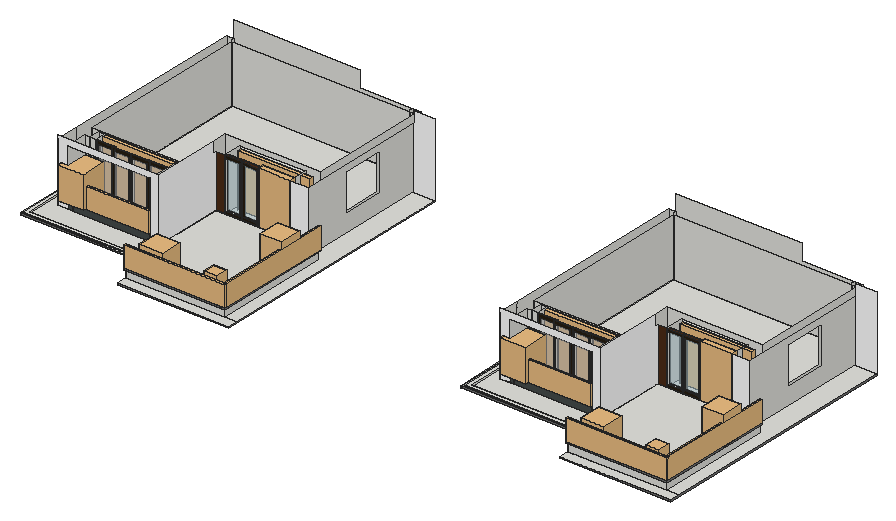
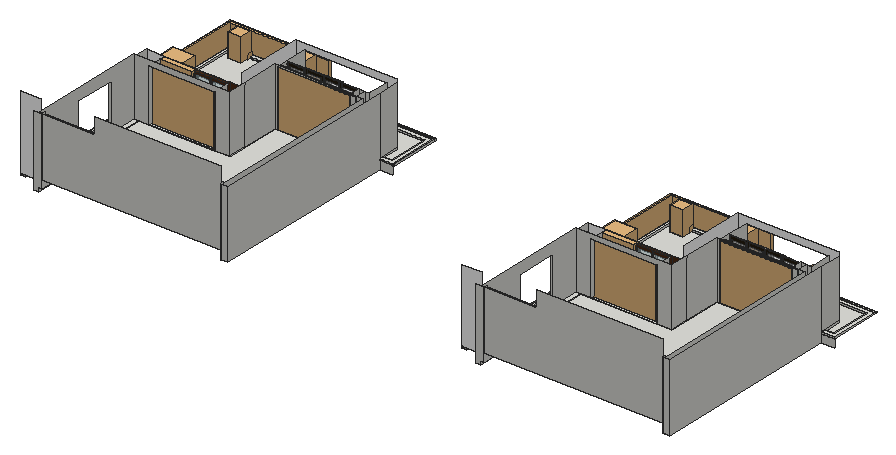
# SketchUp Ruby script. Lengths in inches.
U = 1.inch
M = Sketchup.active_model
def pt(a) = Geom::Point3d.new(a.map { |v| v * U })
def face(e, loops, mat)
  f = e.add_face(loops[0].map { |a| pt(a) })
  loops[1..].each { |l| e.add_face(l.map { |a| pt(a) }).erase! }
  f.material = f.back_material = mat if mat
  f
end
# faces: each face lists its corners as indices into pts; further lists are holes
def faces(e, pts, list, mat = nil) = list.each { |f| face(e, (f[0].is_a?(Array) ? f : [f]).map { |l| l.map { |i| pts[i] } }, mat) }
# xy, xz, yz: faces in a plane at the given z, y or x. An outline is a flat list of corners, or four numbers for a rectangle; further outlines are holes
def ring(l) = l.size == 4 ? [[l[0], l[1]], [l[2], l[1]], [l[2], l[3]], [l[0], l[3]]] : l.each_slice(2).to_a
def flat(e, list, mat, &to3) = list.each { |f| face(e, (f[0].is_a?(Array) ? f : [f]).map { |l| ring(l).map { |u, v| to3.(u, v) } }, mat) }
def xy(e, z, list, mat = nil) = flat(e, list, mat) { |x, y| [x, y, z] }
def xz(e, y, list, mat = nil) = flat(e, list, mat) { |x, z| [x, y, z] }
def yz(e, x, list, mat = nil) = flat(e, list, mat) { |y, z| [x, y, z] }
def lines(e, pts, list) = list.each { |a, b| e.add_line(pt(pts[a]), pt(pts[b])) }
# prism: a flat outline (further loops are holes) pulled along v
def prism(e, loops, v, mat = nil)
  f = face(e, loops, mat); d = Geom::Vector3d.new(v.map { |x| x * U })
  f.pushpull(f.normal.samedirection?(d) ? d.length : -d.length)
end
def box(e, o, s, mat = nil) = prism(e, [[o, [o[0] + s[0], o[1], o[2]], [o[0] + s[0], o[1] + s[1], o[2]], [o[0], o[1] + s[1], o[2]]]], [0, 0, s[2]], mat)
def at(x, y, z, deg = 0) = Geom::Transformation.translation(pt([x, y, z])) * Geom::Transformation.rotation(ORIGIN, Z_AXIS, deg.degrees)
def axes(o, x, y, z) = Geom::Transformation.new([*x, 0, *y, 0, *z, 0, *pt(o).to_a, 1])
def part(name) = M.definitions.add(name)
# library, detail: a bought-in or finely detailed component or shape, given as its bounding box
def library(name, o, s) = part(name).tap { |d| box(d.entities, o, s) }
def detail(e, o, s) = box(e.add_group.entities, o, s)
def put(e, d, t, mat = nil) = e.add_instance(d, t).tap { |i| i.material = mat if mat }
def group(e, t, mat = nil) = e.add_group.tap { |g| g.transformation = t; g.material = mat if mat }.entities
root = M.entities
M.materials.add("[Color M00]").color = [255, 255, 255]
M.materials.add("[Color M05]").color = [114, 114, 114]
M.materials.add("[Slate]").color = [70, 76, 75]
M.materials.add("[Translucent Glass Gray]2").color = [201, 201, 201]
M.materials["[Translucent Glass Gray]2"].alpha = 0.5
M.materials.add("[Translucent Glass Safety]").color = [204, 235, 244]
M.materials["[Translucent Glass Safety]"].alpha = 0.5
M.materials.add("[Wood Veneer 01]").color = [76, 44, 23]
M.materials.add("oak swatch").color = [40, 31, 19]
c1 = library("Glass Railing",[0,0,0],[139.5,4.76,42])
c2 = library("Plant",[0,0,0],[12.59,12.59,14.16])
c3 = library("plant1",[-367.84,-375.82,-125.45],[750.59,696.16,1346.74])
c4 = part("skp4FF")
put(c4.entities,c3,at(0,0,0))
c5 = library("Flora+17",[-57.52,158.6,-38.64],[66.99,62.88,77.28])
c6 = library("plant (1)",[-35.72,-28.42,0],[66.31,67.39,84.38])
c7 = part("Group\#6")
box(c7.entities,[0,0,0],[1.77,4.72,80.31],"oak swatch")
c8 = part("Exterior Sliding Doors")
xy(c8.entities,0,[[1.77,33.07,3.54,70.87],[1.77,70.87,3.54,108.66]])
xy(c8.entities,0,[[0,0,1.77,33.07],[0,108.66,1.77,141.73]],"oak swatch")
xy(c8.entities,4.72,[[0,4.72,1.77,33.07],[1.77,37.8,3.54,66.14],[1.77,75.88,3.54,103.9375],[0,108.66,1.77,137.01]],"oak swatch")
xy(c8.entities,75.59,[[1.77,37.8,3.54,66.14],[1.77,75.88,3.54,103.9375]])
xy(c8.entities,75.59,[[0,4.72,1.77,33.07],[0,108.66,1.77,137.01]],"oak swatch")
xy(c8.entities,80.31,[[0,0,1.77,33.07],[1.77,33.07,3.54,70.87],[1.77,70.87,3.54,108.66],[0,108.66,1.77,141.73]],"oak swatch")
xz(c8.entities,0,[[0,0,1.77,80.31]],"oak swatch")
xz(c8.entities,4.72,[[0,4.72,1.77,75.59]],"oak swatch")
xz(c8.entities,33.07,[[0,0,1.77,4.72],[1.77,0,3.54,80.31],[0,75.59,1.77,80.31]],"oak swatch")
xz(c8.entities,37.8,[[1.77,4.72,3.54,75.59]])
xz(c8.entities,66.14,[[1.77,4.72,3.54,75.59]],"oak swatch")
xz(c8.entities,70.87,[[1.77,0,3.54,80.31]])
xz(c8.entities,75.88,[[1.77,4.72,3.54,75.59]])
xz(c8.entities,103.9375,[[1.77,4.72,3.54,75.59]],"oak swatch")
xz(c8.entities,108.66,[[1.77,4.72,3.54,75.59]])
xz(c8.entities,108.66,[[0,0,3.54,4.72],[0,75.59,3.54,80.31]],"oak swatch")
xz(c8.entities,137.01,[[0,4.72,1.77,75.59]],"oak swatch")
xz(c8.entities,141.73,[[0,0,1.77,80.31]],"oak swatch")
yz(c8.entities,0,[[0,0,33.07,0,33.07,4.72,4.72,4.72,4.72,75.59,33.07,75.59,33.07,80.31,0,80.31],[108.66,0,141.73,0,141.73,80.31,108.66,80.31,108.66,75.59,137.01,75.59,137.01,4.72,108.66,4.72]],"oak swatch")
yz(c8.entities,1.77,[[4.72,4.72,33.07,75.59],[37.8,4.72,66.14,75.59],[75.88,4.72,103.9375,75.59],[108.66,4.72,137.01,75.59]],"[Translucent Glass Gray]2")
yz(c8.entities,1.77,[[0,0,33.07,0,33.07,4.72,4.72,4.72,4.72,75.59,33.07,75.59,33.07,80.31,0,80.31],[[33.07,0,70.87,80.31],[37.8,4.72,66.14,75.59]],[[70.87,0,141.73,80.31],[108.66,4.72,137.01,75.59],[75.88,4.72,103.9375,75.59]]],"oak swatch")
yz(c8.entities,3.54,[[[33.07,0,70.87,80.31],[37.8,4.72,66.14,75.59]],[[70.87,0,108.66,80.31],[75.88,4.72,103.9375,75.59]]],"oak swatch")
put(c8.entities,c7,at(0,33.07,0))
put(c8.entities,c7,at(0,103.9375,0))
c9 = library("Group\#21",[-0.5,-0.5,-0.1],[115.36,88.99,0.2])
c10 = library("Curtains",[0,0,0],[121.73,8.19,117.22])
c11 = part("Group\#4")
g1 = group(c11.entities,at(0,0,0))
xy(g1,0,[[0,0,6,48]],"[Wood Veneer 01]")
xy(g1,4,[[0,4,1.8125,44],[1.8125,4,6,44]])
xy(g1,80,[[0,4,1.8125,44],[1.8125,4,6,44]])
xy(g1,84,[[0,0,6,48]],"[Wood Veneer 01]")
xz(g1,0,[[0,0,6,84]],"[Wood Veneer 01]")
xz(g1,4,[[0,4,1.8125,80],[1.8125,4,6,80]])
xz(g1,44,[[0,4,1.8125,80],[1.8125,4,6,80]])
xz(g1,48,[[0,0,6,84]],"[Wood Veneer 01]")
yz(g1,0,[[[0,0,48,84],[4,4,44,80]]],"[Wood Veneer 01]")
yz(g1,1.8125,[[4,4,44,80]],"[Translucent Glass Safety]")
yz(g1,6,[[[0,0,48,84],[4,4,44,80]]],"oak swatch")
g2 = group(c11.entities,at(0,48,0),"oak swatch")
xy(g2,0,[[0,0,6,48]],"[Wood Veneer 01]")
xy(g2,4,[[0,4,1.8125,44],[1.8125,4,6,44]])
xy(g2,80,[[0,4,1.8125,44],[1.8125,4,6,44]])
xy(g2,84,[[0,0,6,48]],"[Wood Veneer 01]")
xz(g2,0,[[0,0,6,84]],"[Wood Veneer 01]")
xz(g2,4,[[0,4,1.8125,80],[1.8125,4,6,80]])
xz(g2,44,[[0,4,1.8125,80],[1.8125,4,6,80]])
xz(g2,48,[[0,0,6,84]],"[Wood Veneer 01]")
yz(g2,0,[[[0,0,48,84],[4,4,44,80]]],"[Wood Veneer 01]")
yz(g2,1.8125,[[4,4,44,80]],"[Translucent Glass Safety]")
yz(g2,6,[[[0,0,48,84],[4,4,44,80]]],"oak swatch")
c12 = library("modern+door",[0,0,0],[59.06,11.8125,86.61])
xy(root,119.75,[[2097.23,1636.04,2269.48,1636.04,2269.48,1735.1,2276.89,1735.1,2276.89,1746.92,2456.54,1746.92,2456.54,2018.36,2447.32,2018.36,2447.32,1810.9,2440.84,1810.9,2440.84,1773.67,2266.54,1773.67,2266.54,1645.27,2097.23,1645.27],[2989.82,1636.04,3162.07,1636.04,3162.07,1735.1,3169.48,1735.1,3169.48,1746.92,3349.13,1746.92,3349.13,2018.36,3339.91,2018.36,3339.91,1810.9,3333.43,1810.9,3333.43,1773.67,3159.13,1773.67,3159.13,1645.27,2989.82,1645.27]])
xy(root,122.875,[[2276.89,1478.85,2500.29,1488.17],[3169.48,1478.85,3392.88,1488.17],[2489.98,1488.17,2500.29,1998.71],[3382.57,1488.17,3392.88,1998.71]],"[Color M05]")
xy(root,126,[[2276.89,1478.85,2500.29,1499.29],[3169.48,1478.85,3392.88,1499.29],[2276.89,1499.29,2475.98,1535.54],[2475.98,1499.29,2500.29,1499.29,2500.29,1998.71,2456.54,1998.71,2456.54,1735.1,2475.98,1735.1],[3169.48,1499.29,3368.57,1535.54],
  [3368.57,1499.29,3392.88,1499.29,3392.88,1998.71,3349.13,1998.71,3349.13,1735.1,3368.57,1735.1],[2276.89,1535.54,2475.98,1636.04],[3169.48,1535.54,3368.57,1636.04],[2064.92,1636.04,2064.92,2018.36,2079.65,2018.36,2079.65,1659.57,2097.23,1659.57,2097.23,1636.04],[2276.89,1636.04,2475.98,1735.1],
  [2957.51,1636.04,2957.51,2018.36,2972.24,2018.36,2972.24,1659.57,2989.82,1659.57,2989.82,1636.04],[3169.48,1636.04,3368.57,1735.1],[2097.23,1645.27,2097.23,1659.57,2256.86,1659.57,2256.86,1773.67,2266.54,1773.67,2266.54,1645.27],[2989.82,1645.27,2989.82,1659.57,3149.44,1659.57,3149.44,1773.67,3159.13,1773.67,3159.13,1645.27],[2276.89,1735.1,2456.54,1746.92],
  [3169.48,1735.1,3349.13,1746.92],[2440.84,1810.9,2447.32,2018.36],[3333.43,1810.9,3339.91,2018.36]])
xy(root,142.875,[[2276.89,1494.6,2475.98,1499.29],[2475.98,1494.6,2480.67,1499.29],[3169.48,1494.6,3368.57,1499.29],[3368.57,1494.6,3373.26,1499.29],[2276.89,1499.29,2276.89,1535.54,2037.92,1535.54,2037.92,1636.04,2064.92,1636.04,2064.92,1627.67,2046.17,1627.67,2046.17,1544.17,2283.23,1544.17,2283.23,1507.1,2469.67,1507.1,2469.67,1721.3,2456.54,1721.3,2456.54,1735.1,2475.98,1735.1,2475.98,1499.29],
  [2475.98,1499.29,2480.67,1735.1],[3169.48,1499.29,3169.48,1535.54,2930.51,1535.54,2930.51,1636.04,2957.51,1636.04,2957.51,1627.67,2938.76,1627.67,2938.76,1544.17,3175.82,1544.17,3175.82,1507.1,3362.26,1507.1,3362.26,1721.3,3349.13,1721.3,3349.13,1735.1,3368.57,1735.1,3368.57,1499.29],[3368.57,1499.29,3373.26,1735.1],[2283.23,1507.1,2469.67,1507.1,2469.67,1721.3,2456.54,1721.3,2456.54,1735.1,2269.48,1735.1,2269.48,1592.1,2064.92,1592.1,2064.92,1627.67,2046.17,1627.67,2046.17,1544.17,2283.23,1544.17],[3175.82,1507.1,3362.26,1507.1,3362.26,1721.3,3349.13,1721.3,3349.13,1735.1,3162.07,1735.1,3162.07,1592.1,2957.51,1592.1,2957.51,1627.67,2938.76,1627.67,2938.76,1544.17,3175.82,1544.17],
  [2037.92,1530.85,2276.89,1535.54],[2927.19,1530.85,2930.51,1535.54],[2930.51,1530.85,3169.48,1535.54],[2927.19,1535.54,2930.32,1636.04],[2930.32,1535.54,2930.51,1636.04],
  [2064.92,1592.1,2094.14,1592.1,2094.14,1603.46,2084.76,1603.46,2084.76,1636.04,2064.92,1636.04],[2251.32,1592.1,2269.48,1636.04],[2957.51,1592.1,2986.73,1592.1,2986.73,1603.46,2977.35,1603.46,2977.35,1636.04,2957.51,1636.04],[3143.91,1592.1,3162.07,1636.04],[2084.76,1603.46,2251.32,1636.04],
  [2977.35,1603.46,3143.91,1636.04],[2094.14,1636.04,2106.51,1659.57],[2106.51,1636.04,2251.32,1659.57],[2986.73,1636.04,2999.1,1659.57],[2999.1,1636.04,3143.91,1659.57],
  [2079.65,1659.57,2256.86,1659.57,2256.86,1773.67,2440.84,1773.67,2440.84,2011.98,2079.65,2011.98],[2972.24,1659.57,3149.44,1659.57,3149.44,1773.67,3333.43,1773.67,3333.43,2011.98,2972.24,2011.98],[2287.52,1735.1,2419.84,1773.67],[3180.11,1735.1,3312.43,1773.67],[2440.84,1773.67,2450.84,2011.98],
  [3333.43,1773.67,3343.43,2011.98],[2079.65,2011.98,2440.84,2018.36],[2972.24,2011.98,3333.43,2018.36]])
xy(root,146.125,[[2276.89,1494.6,2480.67,1494.6,2480.67,1735.1,2475.98,1735.1,2475.98,1499.29,2276.89,1499.29],[3169.48,1494.6,3373.26,1494.6,3373.26,1735.1,3368.57,1735.1,3368.57,1499.29,3169.48,1499.29],[2276.89,1499.29,2475.98,1499.29,2475.98,1735.1,2456.54,1735.1,2456.54,1721.3,2469.67,1721.3,2469.67,1507.1,2283.23,1507.1,2283.23,1544.17,2046.17,1544.17,2046.17,1627.67,2064.92,1627.67,2064.92,1636.04,2037.92,1636.04,2037.92,1535.54,2276.89,1535.54],[3169.48,1499.29,3368.57,1499.29,3368.57,1735.1,3349.13,1735.1,3349.13,1721.3,3362.26,1721.3,3362.26,1507.1,3175.82,1507.1,3175.82,1544.17,2938.76,1544.17,2938.76,1627.67,2957.51,1627.67,2957.51,1636.04,2930.51,1636.04,2930.51,1535.54,3169.48,1535.54],[2037.92,1530.85,2276.89,1535.54],
  [2927.19,1530.85,2930.51,1535.54],[2930.51,1530.85,3169.48,1535.54],[2927.19,1535.54,2930.32,1636.04],[2930.32,1535.54,2930.51,1636.04]])
xy(root,156.6875,[[2084.76,1592.1,2094.14,1603.46],[2094.14,1592.1,2251.32,1603.46],[2977.35,1592.1,2986.73,1603.46],[2986.73,1592.1,3143.91,1603.46]],"[Slate]")
xz(root,1478.85,[[3169.48,122.875,3392.88,126]],"[Color M05]")
xz(root,1494.6,[[2276.89,142.875,2480.67,146.125],[3169.48,142.875,3373.26,146.125]],"[Color M05]")
xz(root,1499.29,[[2276.89,126,2475.98,142.875],[3169.48,126,3368.57,142.875],[2276.89,142.875,2475.98,146.125],[3169.48,142.875,3368.57,146.125]])
xz(root,1507.1,[[2283.23,142.875,2469.67,146.125],[3175.82,142.875,3362.26,146.125]])
xz(root,1530.85,[[2927.19,142.875,2930.51,146.125]])
xz(root,1530.85,[[2037.92,142.875,2276.89,146.125],[2930.51,142.875,3169.48,146.125]],"[Color M05]")
xz(root,1535.54,[[2037.92,142.875,2276.89,146.125],[2927.19,142.875,2930.32,146.125],[2930.32,142.875,2930.51,146.125],[2930.51,142.875,3169.48,146.125]])
xz(root,1544.17,[[2046.17,142.875,2283.23,146.125],[2938.76,142.875,3175.82,146.125]])
xz(root,1592.1,[[2064.92,142.875,2084.76,142.875,2084.76,257.1875,2251.32,257.1875,2251.32,142.875,2269.48,142.875,2269.48,270.375,2064.92,270.375],[2957.51,142.875,2977.35,142.875,2977.35,257.1875,3143.91,257.1875,3143.91,142.875,3162.07,142.875,3162.07,270.375,2957.51,270.375]],"[Color M00]")
xz(root,1592.1,[[2084.76,142.875,2094.14,156.6875],[2094.14,142.875,2251.32,156.6875],[2977.35,142.875,2986.73,156.6875],[2986.73,142.875,3143.91,156.6875]],"[Slate]")
xz(root,1603.46,[[2084.76,142.875,2094.14,156.6875],[2094.14,142.875,2251.32,156.6875],[2977.35,142.875,2986.73,156.6875],[2986.73,142.875,3143.91,156.6875]])
xz(root,1627.67,[[2046.17,142.875,2064.92,146.125],[2938.76,142.875,2957.51,146.125]])
xz(root,1636.04,[[2097.23,119.75,2269.48,119.75,2269.48,142.875,2064.92,142.875,2064.92,126,2097.23,126],[2989.82,119.75,3162.07,119.75,3162.07,142.875,2957.51,142.875,2957.51,126,2989.82,126],[2037.92,126,2064.92,142.875],[2930.51,126,2957.51,142.875],[2037.92,142.875,2064.92,146.125],
  [2084.76,142.875,2094.14,257.1875],[2094.14,142.875,2106.51,257.1875],[2927.19,142.875,2930.32,146.125],[2930.32,142.875,2930.51,146.125],[2930.51,142.875,2957.51,146.125],
  [2977.35,142.875,2986.73,257.1875],[2986.73,142.875,2999.1,257.1875]])
xz(root,1645.27,[[2097.23,119.75,2266.54,126],[2989.82,119.75,3159.13,126]])
xz(root,1659.57,[[2079.65,126,2256.86,142.875],[2972.24,126,3149.44,142.875],[2079.65,142.875,2079.65,259.3125,2256.86,259.3125,2256.86,142.875,2251.32,142.875,2251.32,257.1875,2094.14,257.1875,2094.14,142.875],[2094.14,142.875,2106.51,257.1875],[2972.24,142.875,2972.24,259.3125,3149.44,259.3125,3149.44,142.875,3143.91,142.875,3143.91,257.1875,2986.73,257.1875,2986.73,142.875],
  [2986.73,142.875,2999.1,257.1875]])
xz(root,1721.3,[[2456.54,142.875,2469.67,146.125],[3349.13,142.875,3362.26,146.125]])
xz(root,1735.1,[[2269.48,119.75,2276.89,119.75,2276.89,126,2456.54,126,2456.54,142.875,2269.48,142.875],[3162.07,119.75,3169.48,119.75,3169.48,126,3349.13,126,3349.13,142.875,3162.07,142.875],[2456.54,126,2475.98,142.875],[3349.13,126,3368.57,142.875],[2456.54,142.875,2475.98,146.125],
  [2475.98,142.875,2480.67,146.125],[3349.13,142.875,3368.57,146.125],[3368.57,142.875,3373.26,146.125]])
xz(root,1735.1,[[2419.84,142.875,2456.54,249.4375],[3312.43,142.875,3349.13,249.4375]],"[Color M00]")
xz(root,1735.1,[[2269.48,142.875,2287.52,249.4375],[3162.07,142.875,3180.11,249.4375]],"[Wood Veneer 01]")
xz(root,1746.92,[[2276.89,119.75,2456.54,126],[3169.48,119.75,3349.13,126]])
xz(root,1773.67,[[2266.54,119.75,2440.84,119.75,2440.84,142.875,2256.86,142.875,2256.86,126,2266.54,126],[3159.13,119.75,3333.43,119.75,3333.43,142.875,3149.44,142.875,3149.44,126,3159.13,126],[2256.86,142.875,2256.86,259.3125,2450.84,259.3125,2450.84,142.875,2419.84,142.875,2419.84,249.4375,2287.52,249.4375,2287.52,142.875],[3149.44,142.875,3149.44,259.3125,3343.43,259.3125,3343.43,142.875,3312.43,142.875,3312.43,249.4375,3180.11,249.4375,3180.11,142.875]])
xz(root,1810.9,[[2440.84,119.75,2447.32,126],[3333.43,119.75,3339.91,126]])
xz(root,1998.71,[[2456.54,126,2500.29,126,2500.29,274.0625,2459.67,274.0625,2459.67,249.4375,2456.54,249.4375],[3349.13,126,3392.88,126,3392.88,274.0625,3352.26,274.0625,3352.26,249.4375,3349.13,249.4375]],"[Color M00]")
xz(root,2011.98,[[2079.65,142.875,2440.84,259.3125],[2440.84,142.875,2450.84,259.3125],[2972.24,142.875,3333.43,259.3125],[3333.43,142.875,3343.43,259.3125]])
xz(root,2018.36,[[2447.32,119.75,2447.32,126,2440.84,126,2440.84,262.875,2456.54,262.875,2456.54,119.75],[3339.91,119.75,3339.91,126,3333.43,126,3333.43,262.875,3349.13,262.875,3349.13,119.75],[2064.92,126,2079.65,262.875],[2957.51,126,2972.24,262.875],[2079.65,142.875,2079.65,295.8125,2333.29,295.8125,2333.29,262.875,2440.84,262.875,2440.84,142.875],
  [2972.24,142.875,2972.24,295.8125,3225.88,295.8125,3225.88,262.875,3333.43,262.875,3333.43,142.875]])
yz(root,2037.92,[[1530.85,142.875,1535.54,146.125],[1535.54,142.875,1636.04,146.125]])
yz(root,2046.17,[[1544.17,142.875,1627.67,146.125]])
yz(root,2064.92,[[1636.04,126,2018.36,262.875],[1592.1,142.875,1627.67,146.125],[1627.67,142.875,1636.04,146.125],[1592.1,146.125,1636.04,262.875]])
yz(root,2079.65,[[1659.57,126,2018.36,142.875],[1659.57,142.875,2011.98,259.3125],[2011.98,142.875,2018.36,262.875]])
yz(root,2084.76,[[1603.46,142.875,1636.04,142.875,1636.04,257.1875,1592.1,257.1875,1592.1,156.6875,1603.46,156.6875]])
yz(root,2094.14,[[1592.1,142.875,1603.46,156.6875],[1636.04,142.875,1659.57,257.1875]])
yz(root,2097.23,[[1636.04,119.75,1645.27,126]])
yz(root,2106.51,[[1636.04,142.875,1659.57,257.1875]])
yz(root,2251.32,[[1592.1,142.875,1603.46,156.6875],[1603.46,142.875,1603.46,156.6875,1592.1,156.6875,1592.1,257.1875,1636.04,257.1875,1636.04,142.875],[1636.04,142.875,1659.57,257.1875]])
yz(root,2256.86,[[1659.57,126,1735.1,142.875],[1735.1,126,1773.67,142.875],[1659.57,142.875,1735.1,259.3125],[1735.1,142.875,1773.67,259.3125]])
yz(root,2266.54,[[1645.27,119.75,1773.67,126]])
yz(root,2269.48,[[1636.04,119.75,1735.1,142.875]])
yz(root,2269.48,[[1592.1,142.875,1735.1,142.875,1735.1,249.4375,1728.29,249.4375,1728.29,270.375,1592.1,270.375]],"[Color M00]")
yz(root,2276.89,[[1735.1,119.75,1746.92,126],[1499.29,126,1535.54,142.875],[1494.6,142.875,1499.29,146.125],[1499.29,142.875,1530.85,146.125],[1530.85,142.875,1535.54,146.125]])
yz(root,2283.23,[[1507.1,142.875,1544.17,146.125]])
yz(root,2287.52,[[1735.1,142.875,1773.67,249.4375]])
yz(root,2419.84,[[1735.1,142.875,1773.67,249.4375]])
yz(root,2440.84,[[1773.67,119.75,1810.9,119.75,1810.9,126,2018.36,126,2018.36,142.875,1773.67,142.875],[2011.98,142.875,2018.36,262.875]])
yz(root,2447.32,[[1810.9,119.75,2018.36,126]])
yz(root,2450.84,[[[1773.67,142.875,2011.98,259.3125],[1830.62,160.58,1916.18,236.83]]])
yz(root,2456.54,[[[1735.1,126,1998.71,249.4375],[1830.62,160.58,1916.18,236.83]],[1721.3,142.875,1735.1,146.125]])
yz(root,2469.67,[[1507.1,142.875,1721.3,146.125]])
yz(root,2475.98,[[1499.29,126,1735.1,142.875],[1499.29,142.875,1735.1,146.125]])
yz(root,2480.67,[[1494.6,142.875,1735.1,146.125]],"[Color M05]")
yz(root,2500.29,[[1478.85,122.875,1998.71,126]],"[Color M05]")
yz(root,2927.19,[[1530.85,142.875,1535.54,146.125],[1535.54,142.875,1636.04,146.125]])
yz(root,2930.32,[[1535.54,142.875,1636.04,146.125]])
yz(root,2930.51,[[1530.85,142.875,1535.54,146.125],[1535.54,142.875,1636.04,146.125]])
yz(root,2938.76,[[1544.17,142.875,1627.67,146.125]])
yz(root,2957.51,[[1636.04,126,2018.36,262.875],[1592.1,142.875,1627.67,146.125],[1627.67,142.875,1636.04,146.125],[1592.1,146.125,1636.04,262.875]])
yz(root,2972.24,[[1659.57,126,2018.36,142.875],[1659.57,142.875,2011.98,259.3125],[2011.98,142.875,2018.36,262.875]])
yz(root,2977.35,[[1603.46,142.875,1636.04,142.875,1636.04,257.1875,1592.1,257.1875,1592.1,156.6875,1603.46,156.6875]])
yz(root,2986.73,[[1592.1,142.875,1603.46,156.6875],[1636.04,142.875,1659.57,257.1875]])
yz(root,2989.82,[[1636.04,119.75,1645.27,126]])
yz(root,2999.1,[[1636.04,142.875,1659.57,257.1875]])
yz(root,3143.91,[[1592.1,142.875,1603.46,156.6875],[1603.46,142.875,1603.46,156.6875,1592.1,156.6875,1592.1,257.1875,1636.04,257.1875,1636.04,142.875],[1636.04,142.875,1659.57,257.1875]])
yz(root,3149.44,[[1659.57,126,1735.1,142.875],[1735.1,126,1773.67,142.875],[1659.57,142.875,1735.1,259.3125],[1735.1,142.875,1773.67,259.3125]])
yz(root,3159.13,[[1645.27,119.75,1773.67,126]])
yz(root,3162.07,[[1636.04,119.75,1735.1,142.875]])
yz(root,3162.07,[[1592.1,142.875,1735.1,142.875,1735.1,249.4375,1728.29,249.4375,1728.29,270.375,1592.1,270.375]],"[Color M00]")
yz(root,3169.48,[[1735.1,119.75,1746.92,126],[1499.29,126,1535.54,142.875],[1494.6,142.875,1499.29,146.125],[1499.29,142.875,1530.85,146.125],[1530.85,142.875,1535.54,146.125]])
yz(root,3175.82,[[1507.1,142.875,1544.17,146.125]])
yz(root,3180.11,[[1735.1,142.875,1773.67,249.4375]])
yz(root,3312.43,[[1735.1,142.875,1773.67,249.4375]])
yz(root,3333.43,[[1773.67,119.75,1810.9,119.75,1810.9,126,2018.36,126,2018.36,142.875,1773.67,142.875],[2011.98,142.875,2018.36,262.875]])
yz(root,3339.91,[[1810.9,119.75,2018.36,126]])
yz(root,3343.43,[[[1773.67,142.875,2011.98,259.3125],[1830.62,160.58,1916.18,236.83]]])
yz(root,3349.13,[[[1735.1,126,1998.71,249.4375],[1830.62,160.58,1916.18,236.83]],[1721.3,142.875,1735.1,146.125]])
yz(root,3362.26,[[1507.1,142.875,1721.3,146.125]])
yz(root,3368.57,[[1499.29,126,1735.1,142.875],[1499.29,142.875,1735.1,146.125]])
yz(root,3373.26,[[1494.6,142.875,1735.1,146.125]],"[Color M05]")
yz(root,3392.88,[[1478.85,122.875,1998.71,126]],"[Color M05]")
put(root,c1,axes([3169.59,1494.6,146.125],[1.46,0,0],[0,1,0],[0,0,1]))
put(root,c1,axes([2277,1494.6,146.125],[1.46,0,0],[0,1,0],[0,0,1]))
put(root,c2,axes([3322.12,1503.64,142.875],[0.7,0,0],[0,0.7,0],[0,0,0.7]))
put(root,c2,axes([2429.53,1503.64,142.875],[0.7,0,0],[0,0.7,0],[0,0,0.7]))
put(root,c4,axes([3335.6,1517.43,147.31],[0.03534,0,0],[0,0.03534,0],[0,0,0.03534]))
put(root,c4,axes([2443.01,1517.43,147.31],[0.03534,0,0],[0,0.03534,0],[0,0,0.03534]))
put(root,c2,axes([3186.16,1515.12,142.875],[0.7,0,0],[0,0.7,0],[0,0,0.7]))
put(root,c2,axes([2293.57,1515.12,142.875],[0.7,0,0],[0,0.7,0],[0,0,0.7]))
put(root,c5,axes([3232.35,1391.38,165.58],[0.71,0,0],[0,0.71,0],[0,0,0.71]))
put(root,c5,axes([2339.76,1391.38,165.58],[0.71,0,0],[0,0.71,0],[0,0,0.71]))
put(root,c1,axes([2977.35,1589.13,157.48],[1.194,0,0],[0,1,0],[0,0,1]))
put(root,c1,axes([2084.76,1589.13,157.48],[1.194,0,0],[0,1,0],[0,0,1]))
put(root,c6,axes([2992.63,1605.18,158.18],[0.77,0,0],[0,0.77,0],[0,0,0.77]))
put(root,c6,axes([2100.04,1605.18,158.18],[0.77,0,0],[0,0.77,0],[0,0,0.77]))
put(root,c1,axes([3373.33,1497.61,146.09],[0,1.70244,0],[-1,0,0],[0,0,1]))
put(root,c1,axes([2480.74,1497.61,146.09],[0,1.70244,0],[-1,0,0],[0,0,1]))
put(root,c8,axes([3000.08,1637.8125,142.875],[0,-1,0],[0.99858,0,0],[0,0,1.4151]))
put(root,c8,axes([2107.49,1637.8125,142.875],[0,-1,0],[0.99858,0,0],[0,0,1.4151]))
put(root,c9,at(2315.71,1595.24,119.375))
put(root,c9,at(3208.3,1595.24,119.375))
put(root,c10,axes([2105.97,1651.375,142.875],[1.19408,0,0],[0,1,0],[0,0,0.96546]))
put(root,c10,axes([2998.5625,1651.375,142.875],[1.19408,0,0],[0,1,0],[0,0,0.96546]))
put(root,c6,axes([2460.18,1656.14,146.125],[0.67,0,0],[0,0.67,0],[0,0,0.67]))
put(root,c6,axes([3352.77,1656.14,146.125],[0.67,0,0],[0,0.67,0],[0,0,0.67]))
put(root,c11,axes([2287,1741.1,142.875],[0,-1,0],[0.71,0,0],[0,0,1.26]))
put(root,c11,axes([3179.59,1741.1,142.875],[0,-1,0],[0.71,0,0],[0,0,1.26]))
put(root,c12,axes([2355.47,1735.1,142.875],[1.09,0,0],[0,1,0],[0,0,1.23031]))
put(root,c12,axes([3248.06,1735.1,142.875],[1.09,0,0],[0,1,0],[0,0,1.23031]))
put(root,c10,axes([3187.16,1759.59,135.21],[1.19408,0,0],[0,1,0],[0,0,0.96546]))
put(root,c10,axes([2294.57,1759.59,135.21],[1.19408,0,0],[0,1,0],[0,0,0.96546]))
